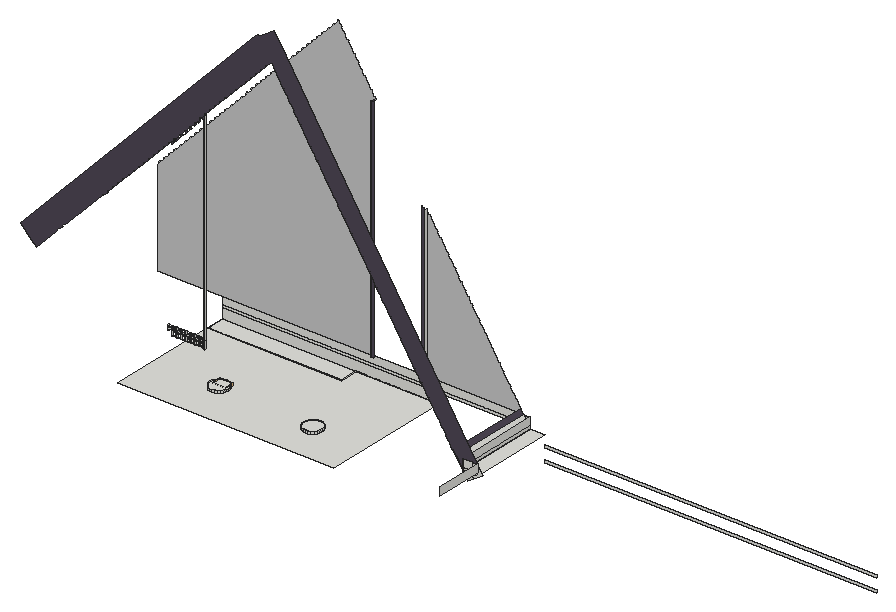
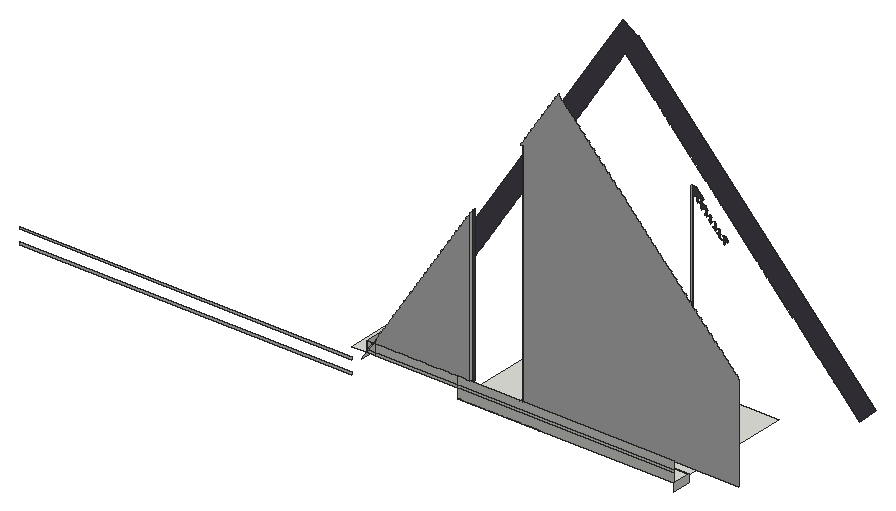
# SketchUp Ruby script. Lengths in inches.
U = 1.inch
M = Sketchup.active_model
def pt(a) = Geom::Point3d.new(a.map { |v| v * U })
def face(e, loops, mat)
  f = e.add_face(loops[0].map { |a| pt(a) })
  loops[1..].each { |l| e.add_face(l.map { |a| pt(a) }).erase! }
  f.material = f.back_material = mat if mat
  f
end
# faces: each face lists its corners as indices into pts; further lists are holes
def faces(e, pts, list, mat = nil) = list.each { |f| face(e, (f[0].is_a?(Array) ? f : [f]).map { |l| l.map { |i| pts[i] } }, mat) }
# xy, xz, yz: faces in a plane at the given z, y or x. An outline is a flat list of corners, or four numbers for a rectangle; further outlines are holes
def ring(l) = l.size == 4 ? [[l[0], l[1]], [l[2], l[1]], [l[2], l[3]], [l[0], l[3]]] : l.each_slice(2).to_a
def flat(e, list, mat, &to3) = list.each { |f| face(e, (f[0].is_a?(Array) ? f : [f]).map { |l| ring(l).map { |u, v| to3.(u, v) } }, mat) }
def xy(e, z, list, mat = nil) = flat(e, list, mat) { |x, y| [x, y, z] }
def xz(e, y, list, mat = nil) = flat(e, list, mat) { |x, z| [x, y, z] }
def yz(e, x, list, mat = nil) = flat(e, list, mat) { |y, z| [x, y, z] }
def lines(e, pts, list) = list.each { |a, b| e.add_line(pt(pts[a]), pt(pts[b])) }
# prism: a flat outline (further loops are holes) pulled along v
def prism(e, loops, v, mat = nil)
  f = face(e, loops, mat); d = Geom::Vector3d.new(v.map { |x| x * U })
  f.pushpull(f.normal.samedirection?(d) ? d.length : -d.length)
end
def box(e, o, s, mat = nil) = prism(e, [[o, [o[0] + s[0], o[1], o[2]], [o[0] + s[0], o[1] + s[1], o[2]], [o[0], o[1] + s[1], o[2]]]], [0, 0, s[2]], mat)
def at(x, y, z, deg = 0) = Geom::Transformation.translation(pt([x, y, z])) * Geom::Transformation.rotation(ORIGIN, Z_AXIS, deg.degrees)
def axes(o, x, y, z) = Geom::Transformation.new([*x, 0, *y, 0, *z, 0, *pt(o).to_a, 1])
def part(name) = M.definitions.add(name)
# library, detail: a bought-in or finely detailed component or shape, given as its bounding box
def library(name, o, s) = part(name).tap { |d| box(d.entities, o, s) }
def detail(e, o, s) = box(e.add_group.entities, o, s)
def put(e, d, t, mat = nil) = e.add_instance(d, t).tap { |i| i.material = mat if mat }
def group(e, t, mat = nil) = e.add_group.tap { |g| g.transformation = t; g.material = mat if mat }.entities
root = M.entities
M.materials.add("[Color M02]").color = [198, 198, 198]
M.materials.add("[Color M06]").color = [79, 71, 84]
c1 = library("A$C06767DEF\#1",[-8.3,1.21,0],[7.09,7.09,5.51])
xy(root,250.875,[[[997.28,2289.06,997.28,2361.68,1083.76,2361.68,1083.76,2373.56,1137.16,2373.56,1137.16,2289.06],[1103.19,2308.39,1104.75,2308.59,1106.19,2309.19,1107.4375,2310.15,1108.39,2311.39,1108.99,2312.84,1109.19,2314.39,1108.99,2315.94,1108.39,2317.39,1107.4375,2318.63,1106.19,2319.58,1104.75,2320.18,1103.19,2320.39,1101.64,2320.18,1100.19,2319.58,1098.95,2318.63,1098,2317.39,1097.4,2315.94,1097.19,2314.39,1097.4,2312.84,1098,2311.39,1098.95,2310.15,1100.19,2309.19,1101.64,2308.59],[1040.12,2311.39,1041.67,2311.59,1043.12,2312.19,1044.36,2313.15,1045.3125,2314.39,1045.91,2315.84,1046.12,2317.39,1045.91,2318.94,1045.3125,2320.39,1044.36,2321.63,1043.12,2322.58,1041.67,2323.18,1040.12,2323.39,1038.5625,2323.18,1037.12,2322.58,1035.875,2321.63,1034.92,2320.39,1034.32,2318.94,1034.12,2317.39,1034.32,2315.84,1034.92,2314.39,1035.875,2313.15,1037.12,2312.19,1038.5625,2311.59]]])
xy(root,251.0625,[[997.28,2361.68,1083.76,2373.56]])
xy(root,252.25,[[1103.19,2308.39,1101.64,2308.59,1100.19,2309.19,1098.95,2310.15,1098,2311.39,1097.4,2312.84,1097.19,2314.39,1097.4,2315.94,1098,2317.39,1098.95,2318.63,1100.19,2319.58,1101.64,2320.18,1103.19,2320.39,1104.75,2320.18,1106.19,2319.58,1107.4375,2318.63,1108.39,2317.39,1108.99,2315.94,1109.19,2314.39,1108.99,2312.84,1108.39,2311.39,1107.4375,2310.15,1106.19,2309.19,1104.75,2308.59]])
xy(root,252.375,[[1040.12,2311.39,1038.5625,2311.59,1037.12,2312.19,1035.875,2313.15,1034.92,2314.39,1034.32,2315.84,1034.12,2317.39,1034.32,2318.94,1034.92,2320.39,1035.875,2321.63,1037.12,2322.58,1038.5625,2323.18,1040.12,2323.39,1041.67,2323.18,1043.12,2322.58,1044.36,2321.63,1045.3125,2320.39,1045.91,2318.94,1046.12,2317.39,1045.91,2315.84,1045.3125,2314.39,1044.36,2313.15,1043.12,2312.19,1041.67,2311.59]])
xy(root,257.0625,[[1196.26,2319.18,1205.57,2373.56]])
xy(root,259.68,[[998.06,2332.13,1000.37,2332.76],[1000.97,2332.13,1003.28,2332.76],[1003.88,2332.13,1006.2,2332.76],[1006.79,2332.13,1009.11,2332.76],[1009.71,2332.13,1012.02,2332.76],
  [1012.62,2332.13,1014.93,2332.76],[1015.53,2332.13,1017.84,2332.76]])
xy(root,262,[[995.15,2332.13,997.46,2332.76],[998.06,2332.13,1000.37,2332.76],[1000.97,2332.13,1003.28,2332.76],[1003.88,2332.13,1006.2,2332.76],[1006.79,2332.13,1009.11,2332.76],
  [1009.71,2332.13,1012.02,2332.76],[1012.62,2332.13,1014.93,2332.76],[1015.53,2332.13,1017.84,2332.76]])
xy(root,262.73,[[995.18,2332.13,997.49,2332.76],[998.09,2332.13,1000.4,2332.76],[1001,2332.13,1003.3125,2332.76],[1003.91,2332.13,1006.22,2332.76],[1006.82,2332.13,1009.14,2332.76],
  [1009.74,2332.13,1012.05,2332.76],[1012.65,2332.13,1014.96,2332.76],[1015.56,2332.13,1017.87,2332.76]])
xy(root,263.89,[[1095.04,2371.68,1096.79,2373.56],[1127.76,2371.68,1129.63,2373.56]])
xy(root,265.04,[[995.18,2332.13,997.49,2332.76],[998.09,2332.13,1000.4,2332.76],[1001,2332.13,1003.3125,2332.76],[1003.91,2332.13,1006.22,2332.76],[1006.82,2332.13,1009.14,2332.76],
  [1009.74,2332.13,1012.05,2332.76],[1012.65,2332.13,1014.96,2332.76],[1015.56,2332.13,1017.87,2332.76]])
xz(root,2319.18,[[1199.5,252.01,1203.55,254.61,1201.98,257.0625,1196.26,257.0625],[1203.55,254.61,1208.8125,257.98,1205.57,263.03,1205.57,257.0625,1201.98,257.0625],[1196.26,257.0625,1201.98,258.95],[1201.98,257.0625,1205.57,258.95],[1196.26,258.95,1201.98,263.89],
  [1201.98,258.95,1205.57,258.95,1205.57,263.03,1205.03,263.89,1201.98,263.89],[1205.57,263.03,1205.03,263.89,1205.57,263.89]])
xz(root,2319.18,[[1196.26,257.0625,1196.26,263.89,1205.03,263.89,1081.6,456.41,1073.92,468.38,1068.66,465.01,1064.27,462.19,1063.71,462.72,1062.38,461.31,910.18,299.61,917.71,292.52,920.85,289.56,923.27,292.13,924.15,293.0625,926.57,295.64,927.45,296.57,929.87,299.14,930.75,300.07,933.17,302.64,934.05,303.58,933.82,303.79,936.24,306.36,936.47,306.15,937.35,307.08,937.12,307.29,939.54,309.87,939.77,309.65,940.64,310.59,943.07,313.16,943.94,314.09,946.36,316.66,947.24,317.59,949.66,320.17,950.54,321.1,952.96,323.67,953.84,324.6,956.26,327.17,957.14,328.11,959.56,330.68,960.4375,331.61,962.86,334.18,963.73,335.11,964.1875,334.6875,966.61,337.26,966.16,337.6875,967.03,338.62,967.49,338.19,969.91,340.76,969.45,341.19,970.33,342.125,970.79,341.69,973.21,344.27,972.75,344.7,973.63,345.63,974.08,345.2,976.51,347.77,976.05,348.2,976.93,349.13,977.38,348.7,979.8,351.28,979.35,351.7,980.23,352.64,980.68,352.21,983.1,354.78,982.65,355.21,983.53,356.14,983.98,355.71,986.4,358.28,985.95,358.71,986.82,359.64,987.28,359.22,989.7,361.79,989.25,362.22,990.12,363.15,990.58,362.72,993,365.29,992.54,365.72,993.42,366.65,993.875,366.22,996.3,368.8,995.84,369.23,996.72,370.16,997.17,369.73,999.6,372.3,999.14,372.73,1000.02,373.66,1000.47,373.23,1002.89,375.81,1002.4375,376.23,1003.32,377.17,1003.77,376.74,1006.19,379.31,1005.74,379.74,1006.62,380.67,1007.07,380.24,1009.49,382.8125,1009.04,383.24,1009.91,384.17,1010.37,383.75,1012.79,386.32,1012.33,386.75,1013.21,387.68,1013.67,387.25,1016.09,389.82,1015.63,390.25,1016.51,391.18,1016.97,390.75,1019.39,393.33,1018.93,393.75,1019.81,394.6875,1020.26,394.26,1022.6875,396.83,1022.23,397.26,1023.11,398.19,1023.5625,397.76,1025.98,400.34,1025.53,400.76,1026.41,401.7,1026.86,401.27,1029.28,403.84,1028.83,404.27,1029.71,405.2,1030.16,404.77,1032.58,407.34,1032.125,407.77,1033,408.7,1033.46,408.28,1035.88,410.85,1035.42,411.28,1036.3,412.21,1036.76,411.78,1039.18,414.35,1038.72,414.78,1039.6,415.71,1040.06,415.28,1042.48,417.86,1042.02,418.28,1042.9,419.22,1043.35,418.79,1045.78,421.36,1045.32,421.79,1046.2,422.72,1046.65,422.29,1049.07,424.86,1048.62,425.29,1049.5,426.23,1049.95,425.8,1052.37,428.37,1051.92,428.8,1052.79,429.73,1053.25,429.3,1055.67,431.875,1055.22,432.3,1056.09,433.23,1056.55,432.81,1058.97,435.38,1058.51,435.81,1059.39,436.74,1059.85,436.31,1062.27,438.88,1061.8125,439.31,1062.69,440.24,1063.15,439.8125,1065.57,442.39,1065.11,442.8125,1065.99,443.75,1066.44,443.32,1068.87,445.89,1068.41,446.32,1069.29,447.25,1069.74,446.82,1072.16,449.39,1071.71,449.82,1071.98,450.11,1071.92,450.2,1072.29,450.4375,1073.86,447.99,1074.35,447.21,1073.99,446.98,1075.68,444.33,1076.05,444.57,1076.55,443.79,1076.18,443.56,1077.875,440.91,1078.24,441.15,1078.74,440.375,1078.37,440.14,1080.07,437.49,1080.43,437.73,1080.93,436.95,1080.5625,436.72,1082.26,434.07,1082.625,434.31,1083.125,433.53,1082.76,433.3,1084.45,430.65,1084.82,430.89,1085.32,430.11,1084.95,429.88,1086.64,427.23,1087.01,427.47,1087.51,426.69,1087.14,426.46,1088.84,423.8125,1089.2,424.05,1089.7,423.27,1089.33,423.04,1091.03,420.39,1091.4,420.63,1091.9,419.85,1091.53,419.62,1093.22,416.97,1093.59,417.21,1094.09,416.43,1093.72,416.2,1095.41,413.55,1095.78,413.79,1096.28,413.01,1095.91,412.78,1097.61,410.13,1097.97,410.37,1098.47,409.59,1098.1,409.36,1099.8,406.71,1100.17,406.95,1100.67,406.17,1100.3,405.9375,1101.99,403.29,1102.36,403.53,1102.86,402.75,1102.49,402.52,1104.18,399.875,1104.55,400.11,1105.05,399.33,1104.68,399.1,1106.375,396.45,1106.75,396.69,1107.24,395.91,1106.875,395.68,1108.57,393.03,1108.9375,393.27,1109.4375,392.49,1109.07,392.26,1110.76,389.61,1111.13,389.85,1111.63,389.07,1111.26,388.84,1112.95,386.19,1113.32,386.43,1113.82,385.65,1113.45,385.42,1115.15,382.77,1115.52,383.01,1116.01,382.23,1115.65,382,1117.34,379.35,1117.71,379.59,1118.21,378.8125,1117.84,378.58,1119.53,375.93,1119.9,376.17,1120.4,375.39,1120.03,375.16,1121.72,372.51,1122.09,372.75,1122.59,371.97,1122.22,371.74,1123.92,369.09,1124.29,369.33,1124.92,368.34,1124.55,368.11,1126.25,365.46,1126.61,365.7,1127.25,364.71,1128.94,362.07,1129.57,361.08,1129.21,360.85,1130.9,358.2,1131.27,358.4375,1131.9,357.45,1131.53,357.22,1133.23,354.57,1133.6,354.81,1134.23,353.82,1133.86,353.58,1135.56,350.94,1135.92,351.18,1136.56,350.19,1136.1875,349.95,1137.88,347.3125,1138.25,347.55,1138.88,346.56,1138.52,346.32,1140.21,343.68,1140.58,343.92,1141.21,342.93,1140.84,342.69,1142.54,340.05,1142.91,340.29,1143.4375,339.46,1143.07,339.22,1144.76,336.58,1145.13,336.8125,1145.66,335.98,1145.3,335.75,1146.99,333.11,1147.36,333.34,1147.89,332.51,1147.52,332.28,1149.22,329.63,1149.59,329.87,1150.12,329.04,1149.75,328.8,1151.44,326.16,1151.8125,326.4,1152.34,325.57,1151.98,325.33,1153.67,322.6875,1154.04,322.92,1154.57,322.09,1154.2,321.86,1155.9,319.21,1156.26,319.45,1156.8,318.62,1156.43,318.38,1158.12,315.74,1158.49,315.98,1159.02,315.15,1158.65,314.91,1160.35,312.27,1160.72,312.51,1161.25,311.68,1160.88,311.44,1162.57,308.8,1162.94,309.03,1163.47,308.2,1163.11,307.97,1164.8,305.32,1165.17,305.56,1165.7,304.73,1165.33,304.49,1167.03,301.85,1167.4,302.09,1167.93,301.26,1167.66,301.09,1169.36,298.45,1169.62,298.61,1170.15,297.79,1169.89,297.62,1171.59,294.97,1171.85,295.14,1172.38,294.3125,1172.12,294.14,1173.8125,291.5,1174.07,291.67,1174.61,290.84,1174.34,290.67,1176.04,288.03,1176.3,288.2,1176.83,287.37,1176.57,287.2,1178.26,284.56,1178.53,284.72,1179.06,283.89,1178.8,283.73,1180.49,281.08,1180.75,281.25,1181.29,280.42,1181.02,280.25,1182.72,277.61,1182.98,277.78,1183.51,276.95,1183.25,276.78,1184.94,274.14,1185.21,274.31,1185.74,273.48,1185.48,273.31,1187.17,270.67,1187.43,270.83,1187.96,270,1187.7,269.84,1189.4,267.19,1189.66,267.36,1190.19,266.53,1189.93,266.36,1191.62,263.72,1191.89,263.89]],"[Color M06]")
xz(root,2332.13,[[1018.44,258.95,1019.02,263.89],[995.18,262.73,997.49,263.89],[998.09,262.73,1000.4,263.89],[1001,262.73,1003.3125,263.89],[1003.91,262.73,1006.22,263.89],
  [1006.82,262.73,1009.14,263.89],[1009.74,262.73,1012.05,263.89],[1012.65,262.73,1014.96,263.89],[1015.56,262.73,1017.87,263.89]])
xz(root,2332.13,[[1018.44,263.89,1019.02,263.89,1019.02,397.75,1016.77,397.75,1011.26,391.9,1012.48,391.9,1012.48,390.44,1013.08,391.08,1013.08,391.9,1015.4,391.9,1015.4,389.59,1013.08,389.59,1013.08,391.08,1012.48,390.44,1012.48,389.59,1011.68,389.59,1011.27,389.15,1010.28,389.15,1010.17,389.03,1010.17,387.98,1009.57,387.35,1009.57,386.84,1009.09,386.84,1008.68,386.4,1009.57,386.4,1009.57,384.09,1007.26,384.09,1007.26,384.89,1006.66,384.25,1006.66,384.09,1006.5,384.09,1006.09,383.65,1006.66,383.65,1006.66,381.34,1004.35,381.34,1004.35,381.8,1003.5,380.9,1003.75,380.9,1003.75,378.59,1001.43,378.59,1001.43,378.7,1000.83,378.07,1000.83,375.84,998.74,375.84,997.92,374.97,997.92,373.09,996.15,373.09,997.92,374.97,997.92,375.4,997.27,375.4,995.61,373.625,995.61,373.09,996.15,373.09,995.68,372.59,997.92,372.59,997.92,370.47,998.52,371.11,998.52,372.59,999.91,372.59,1000.38,373.09,998.52,373.09,998.52,375.4,1000.83,375.4,1000.83,373.57,1001.43,374.21,1001.43,375.4,1002.55,375.4,1002.96,375.84,1001.43,375.84,1001.43,378.15,1003.75,378.15,1003.75,376.68,1004.35,377.32,1004.35,378.15,1005.125,378.15,1005.53,378.59,1004.35,378.59,1004.35,380.9,1006.66,380.9,1006.66,379.79,1007.26,380.43,1007.26,380.9,1007.7,380.9,1008.11,381.34,1007.26,381.34,1007.26,383.65,1009.57,383.65,1009.57,382.89,1010.17,383.53,1010.17,383.65,1010.28,383.65,1010.37,383.75,1010.69,384.09,1010.17,384.09,1010.17,386.4,1012.48,386.4,1012.48,386,1013.27,386.84,1013.08,386.84,1013.08,389.15,1015.4,389.15,1015.4,389.11,1015.99,389.75,1015.99,391.9,1018.01,391.9,1018.44,392.36]],"[Color M06]")
xz(root,2332.76,[[995.18,262.73,997.49,263.89],[998.09,262.73,1000.4,263.89],[1001,262.73,1003.3125,263.89],[1003.91,262.73,1006.22,263.89],[1006.82,262.73,1009.14,263.89],
  [1009.74,262.73,1012.05,263.89],[1012.65,262.73,1014.96,263.89],[1015.56,262.73,1017.87,263.89]])
xz(root,2361.68,[[997.28,250.875,1083.76,251.0625]])
xz(root,2371.68,[[1095.04,263.89,1096.79,412.22],[1127.76,263.89,1129.63,263.89,1129.63,360.99,1129.26,360.76,1129.21,360.85,1129.57,361.08,1128.94,362.07,1128.57,361.83,1127.76,363.11]],"[Color M06]")
xz(root,2373.56,[[1205.57,240.88,1419.96,242.34],[1205.57,249.61,1419.96,251.0625],[1083.76,250.875,1137.16,251.0625],[997.28,251.0625,1137.16,257.0625],[997.28,257.0625,1137.16,258.95],
  [1137.16,257.0625,1190.19,258.95],[1190.19,257.0625,1196.26,257.0625,1195.05,258.95,1190.19,258.95],[1196.26,257.0625,1195.05,258.95,1196.26,258.95],[997.28,258.95,1137.16,263.89],[1137.16,258.95,1190.19,263.89],
  [1190.19,258.95,1195.05,258.95,1191.89,263.89,1191.62,263.72,1191.51,263.89,1190.19,263.89],[1195.05,258.95,1191.89,263.89,1195.05,263.89],[1195.05,258.95,1196.26,263.89],[1191.62,263.72,1191.51,263.89,1191.89,263.89]])
xz(root,2373.56,[[955.23,263.89,1095.04,263.89,1095.04,412.22,1096.27,412.22,1095.97,412.6875,1096.34,412.92,1095.78,413.79,1095.41,413.55,1094.23,415.41,1093.78,416.11,1094.14,416.34,1093.59,417.21,1093.22,416.97,1092.03,418.83,1091.58,419.53,1091.95,419.76,1091.4,420.63,1091.03,420.39,1089.84,422.25,1089.39,422.95,1089.76,423.18,1089.2,424.05,1088.84,423.8125,1087.65,425.67,1087.2,426.37,1087.57,426.6,1087.01,427.47,1086.64,427.23,1085.46,429.09,1085.01,429.79,1085.375,430.02,1084.82,430.89,1084.45,430.65,1083.26,432.51,1082.8125,433.21,1083.18,433.44,1082.625,434.31,1082.26,434.07,1081.07,435.93,1080.62,436.63,1080.99,436.86,1080.43,437.73,1080.07,437.49,1078.88,439.35,1078.43,440.05,1078.8,440.28,1078.24,441.15,1077.875,440.91,1076.69,442.77,1076.24,443.47,1076.6,443.7,1076.05,444.57,1075.68,444.33,1074.49,446.1875,1074.04,446.89,1074.41,447.125,1073.86,447.99,1073.49,447.75,1072.3,449.61,1071.98,450.11,1071.71,449.82,1072.16,449.39,1069.74,446.82,1069.29,447.25,1068.41,446.32,1068.87,445.89,1066.44,443.32,1065.99,443.75,1065.11,442.8125,1065.57,442.39,1063.15,439.8125,1062.69,440.24,1061.8125,439.31,1062.27,438.88,1059.85,436.31,1059.39,436.74,1058.51,435.81,1058.97,435.38,1056.55,432.81,1056.09,433.23,1055.22,432.3,1055.67,431.875,1053.25,429.3,1052.79,429.73,1051.92,428.8,1052.37,428.37,1049.95,425.8,1049.5,426.23,1048.62,425.29,1049.07,424.86,1046.65,422.29,1046.2,422.72,1045.32,421.79,1045.78,421.36,1043.35,418.79,1042.9,419.22,1042.02,418.28,1042.48,417.86,1040.06,415.28,1039.6,415.71,1038.72,414.78,1039.18,414.35,1036.76,411.78,1036.3,412.21,1035.42,411.28,1035.88,410.85,1033.46,408.28,1033,408.7,1032.125,407.77,1032.58,407.34,1030.16,404.77,1029.71,405.2,1028.83,404.27,1029.28,403.84,1026.86,401.27,1026.41,401.7,1025.53,400.76,1025.98,400.34,1023.5625,397.76,1023.11,398.19,1022.23,397.26,1022.6875,396.83,1020.26,394.26,1019.81,394.6875,1018.93,393.75,1019.39,393.33,1016.97,390.75,1016.51,391.18,1015.63,390.25,1016.09,389.82,1013.67,387.25,1013.21,387.68,1012.33,386.75,1012.79,386.32,1010.37,383.75,1009.91,384.17,1009.04,383.24,1009.49,382.8125,1007.07,380.24,1006.62,380.67,1005.74,379.74,1006.19,379.31,1003.77,376.74,1003.32,377.17,1002.4375,376.23,1002.89,375.81,1000.47,373.23,1000.02,373.66,999.14,372.73,999.6,372.3,997.17,369.73,996.72,370.16,995.84,369.23,996.3,368.8,993.875,366.22,993.42,366.65,992.54,365.72,993,365.29,990.58,362.72,990.12,363.15,989.25,362.22,989.7,361.79,987.28,359.22,986.82,359.64,985.95,358.71,986.4,358.28,983.98,355.71,983.53,356.14,982.65,355.21,983.1,354.78,980.68,352.21,980.23,352.64,979.35,351.7,979.8,351.28,977.38,348.7,976.93,349.13,976.05,348.2,976.51,347.77,974.08,345.2,973.63,345.63,972.75,344.7,973.21,344.27,970.79,341.69,970.33,342.125,969.45,341.19,969.91,340.76,969.31,340.125,968.91,339.7,967.49,338.19,967.03,338.62,966.16,337.6875,966.61,337.26,964.1875,334.6875,963.73,335.11,962.86,334.18,963.3125,333.75,960.89,331.18,960.4375,331.61,959.56,330.68,960.01,330.25,957.59,327.68,957.14,328.11,956.26,327.17,956.71,326.75,955.6875,325.65,955.23,325.17],[1129.63,263.89,1190.19,263.89,1190.19,265.95,1189.93,266.36,1190.19,266.53,1189.66,267.36,1189.4,267.19,1187.7,269.84,1187.96,270,1187.43,270.83,1187.17,270.67,1185.48,273.31,1185.74,273.48,1185.21,274.31,1184.94,274.14,1183.25,276.78,1183.51,276.95,1182.98,277.78,1182.72,277.61,1181.02,280.25,1181.29,280.42,1180.75,281.25,1180.49,281.08,1178.8,283.73,1179.06,283.89,1178.53,284.72,1178.26,284.56,1176.57,287.2,1176.83,287.37,1176.3,288.2,1176.04,288.03,1174.34,290.67,1174.61,290.84,1174.07,291.67,1173.8125,291.5,1172.12,294.14,1172.38,294.3125,1171.85,295.14,1171.59,294.97,1169.89,297.62,1170.15,297.79,1169.62,298.61,1169.36,298.45,1167.66,301.09,1167.93,301.26,1167.4,302.09,1167.03,301.85,1165.33,304.49,1165.7,304.73,1165.17,305.56,1164.8,305.32,1163.11,307.97,1163.47,308.2,1162.94,309.03,1162.57,308.8,1160.88,311.44,1161.25,311.68,1160.72,312.51,1160.35,312.27,1158.65,314.91,1159.02,315.15,1158.49,315.98,1158.12,315.74,1156.43,318.38,1156.8,318.62,1156.26,319.45,1155.9,319.21,1154.2,321.86,1154.57,322.09,1154.04,322.92,1153.67,322.6875,1151.98,325.33,1152.34,325.57,1151.8125,326.4,1151.44,326.16,1149.75,328.8,1150.12,329.04,1149.59,329.87,1149.22,329.63,1147.52,332.28,1147.89,332.51,1147.36,333.34,1146.99,333.11,1145.3,335.75,1145.66,335.98,1145.13,336.8125,1144.76,336.58,1143.07,339.22,1143.4375,339.46,1143.01,340.125,1142.91,340.29,1142.54,340.05,1140.84,342.69,1141.21,342.93,1140.58,343.92,1140.21,343.68,1138.52,346.32,1138.88,346.56,1138.25,347.55,1137.88,347.3125,1136.1875,349.95,1136.56,350.19,1135.92,351.18,1135.56,350.94,1133.86,353.58,1134.23,353.82,1133.6,354.81,1133.23,354.57,1131.53,357.22,1131.9,357.45,1131.27,358.4375,1130.9,358.2,1129.63,360.18]],"[Color M02]")
yz(root,997.28,[[2361.68,246.25,2373.56,251.0625]])
yz(root,997.46,[[2332.13,259.68,2332.76,262]])
yz(root,997.49,[[2332.13,262.73,2332.76,265.04]])
yz(root,998.06,[[2332.13,259.68,2332.76,262]])
yz(root,998.09,[[2332.13,262.73,2332.76,265.04]])
yz(root,1000.37,[[2332.13,259.68,2332.76,262]])
yz(root,1000.4,[[2332.13,262.73,2332.76,265.04]])
yz(root,1000.97,[[2332.13,259.68,2332.76,262]])
yz(root,1001,[[2332.13,262.73,2332.76,265.04]])
yz(root,1003.28,[[2332.13,259.68,2332.76,262]])
yz(root,1003.3125,[[2332.13,262.73,2332.76,265.04]])
yz(root,1003.88,[[2332.13,259.68,2332.76,262]])
yz(root,1003.91,[[2332.13,262.73,2332.76,265.04]])
yz(root,1006.2,[[2332.13,259.68,2332.76,262]])
yz(root,1006.22,[[2332.13,262.73,2332.76,265.04]])
yz(root,1006.79,[[2332.13,259.68,2332.76,262]])
yz(root,1006.82,[[2332.13,262.73,2332.76,265.04]])
yz(root,1009.11,[[2332.13,259.68,2332.76,262]])
yz(root,1009.14,[[2332.13,262.73,2332.76,265.04]])
yz(root,1009.71,[[2332.13,259.68,2332.76,262]])
yz(root,1009.74,[[2332.13,262.73,2332.76,265.04]])
yz(root,1012.02,[[2332.13,259.68,2332.76,262]])
yz(root,1012.05,[[2332.13,262.73,2332.76,265.04]])
yz(root,1012.62,[[2332.13,259.68,2332.76,262]])
yz(root,1012.65,[[2332.13,262.73,2332.76,265.04]])
yz(root,1014.93,[[2332.13,259.68,2332.76,262]])
yz(root,1014.96,[[2332.13,262.73,2332.76,265.04]])
yz(root,1015.53,[[2332.13,259.68,2332.76,262]])
yz(root,1015.56,[[2332.13,262.73,2332.76,265.04]])
yz(root,1017.84,[[2332.13,259.68,2332.76,262]])
yz(root,1017.87,[[2332.13,262.73,2332.76,265.04]])
yz(root,1019.02,[[2332.13,258.95,2332.76,263.89],[2332.13,263.89,2332.76,397.75]])
yz(root,1083.76,[[2361.68,250.875,2373.56,251.0625]])
yz(root,1095.04,[[2371.68,263.89,2373.56,412.22]],"[Color M06]")
yz(root,1129.63,[[2371.68,263.89,2373.56,360.99]])
yz(root,1196.26,[[2319.18,257.0625,2373.56,258.95],[2319.18,258.95,2373.56,263.89]])
yz(root,1205.57,[[2289.06,258.95,2319.18,263.89]])
p = [[1103.19,2308.39,250.875],[1101.64,2308.59,250.875],[1101.64,2308.59,252.25],[1103.19,2308.39,252.25],[1104.75,2308.59,250.875],[1104.75,2308.59,252.25],
  [1100.19,2309.19,250.875],[1100.19,2309.19,252.25],[1106.19,2309.19,250.875],[1106.19,2309.19,252.25],[1098.95,2310.15,250.875],[1098.95,2310.15,252.25],
  [1107.4375,2310.15,250.875],[1107.4375,2310.15,252.25],[1098,2311.39,250.875],[1098,2311.39,252.25],[1108.39,2311.39,250.875],[1108.39,2311.39,252.25],
  [1040.12,2311.39,250.875],[1038.5625,2311.59,250.875],[1038.5625,2311.59,252.375],[1040.12,2311.39,252.375],[1041.67,2311.59,250.875],[1041.67,2311.59,252.375],
  [1097.4,2312.84,250.875],[1097.4,2312.84,252.25],[1108.99,2312.84,250.875],[1108.99,2312.84,252.25],[1037.12,2312.19,250.875],[1037.12,2312.19,252.375],
  [1043.12,2312.19,250.875],[1043.12,2312.19,252.375],[1035.875,2313.15,250.875],[1035.875,2313.15,252.375],[1044.36,2313.15,250.875],[1044.36,2313.15,252.375],
  [1097.19,2314.39,250.875],[1097.19,2314.39,252.25],[1109.19,2314.39,250.875],[1109.19,2314.39,252.25],[1034.92,2314.39,250.875],[1034.92,2314.39,252.375],
  [1045.3125,2314.39,250.875],[1045.3125,2314.39,252.375],[1034.32,2315.84,250.875],[1034.32,2315.84,252.375],[1045.91,2315.84,250.875],[1045.91,2315.84,252.375],
  [1097.4,2315.94,250.875],[1097.4,2315.94,252.25],[1108.99,2315.94,250.875],[1108.99,2315.94,252.25],[1034.12,2317.39,250.875],[1034.12,2317.39,252.375],
  [1046.12,2317.39,250.875],[1046.12,2317.39,252.375],[1098,2317.39,250.875],[1098,2317.39,252.25],[1108.39,2317.39,250.875],[1108.39,2317.39,252.25],
  [1034.32,2318.94,250.875],[1034.32,2318.94,252.375],[1045.91,2318.94,250.875],[1045.91,2318.94,252.375],[1098.95,2318.63,250.875],[1098.95,2318.63,252.25],
  [1107.4375,2318.63,250.875],[1107.4375,2318.63,252.25],[1100.19,2319.58,250.875],[1100.19,2319.58,252.25],[1106.19,2319.58,250.875],[1106.19,2319.58,252.25],
  [1034.92,2320.39,250.875],[1034.92,2320.39,252.375],[1045.3125,2320.39,250.875],[1045.3125,2320.39,252.375],[1101.64,2320.18,250.875],[1101.64,2320.18,252.25],
  [1104.75,2320.18,250.875],[1104.75,2320.18,252.25],[1103.19,2320.39,250.875],[1103.19,2320.39,252.25],[1035.875,2321.63,250.875],[1035.875,2321.63,252.375],
  [1044.36,2321.63,250.875],[1044.36,2321.63,252.375],[1037.12,2322.58,250.875],[1037.12,2322.58,252.375],[1043.12,2322.58,250.875],[1043.12,2322.58,252.375],
  [1038.5625,2323.18,250.875],[1038.5625,2323.18,252.375],[1041.67,2323.18,250.875],[1041.67,2323.18,252.375],[1040.12,2323.39,250.875],[1040.12,2323.39,252.375],
  [1196.26,2319.18,257.0625],[1196.26,2373.56,257.0625],[1199.5,2373.56,252.01],[1199.5,2319.18,252.01],[1191.89,2319.18,263.89],[1191.89,2373.56,263.89],
  [1195.05,2373.56,258.95],[1189.93,2373.56,266.36],[1190.19,2373.56,265.95],[1191.51,2373.56,263.89],[1191.62,2373.56,263.72],[1191.62,2319.18,263.72],
  [1189.93,2319.18,266.36]]
faces(root,p,[[0,1,2,3],[4,0,3,5],[1,6,7,2],[8,4,5,9],[6,10,11,7],[12,8,9,13],[10,14,15,11],[16,12,13,17],
  [18,19,20,21],[22,18,21,23],[14,24,25,15],[26,16,17,27],[19,28,29,20],[30,22,23,31],[28,32,33,29],[34,30,31,35],
  [24,36,37,25],[38,26,27,39],[32,40,41,33],[42,34,35,43],[40,44,45,41],[46,42,43,47],[36,48,49,37],[50,38,39,51],
  [44,52,53,45],[54,46,47,55],[48,56,57,49],[58,50,51,59],[52,60,61,53],[62,54,55,63],[56,64,65,57],[66,58,59,67],
  [64,68,69,65],[70,66,67,71],[60,72,73,61],[74,62,63,75],[68,76,77,69],[78,70,71,79],[76,80,81,77],[80,78,79,81],
  [72,82,83,73],[84,74,75,85],[82,86,87,83],[88,84,85,89],[86,90,91,87],[92,88,89,93],[90,94,95,91],[94,92,93,95],
  [96,97,98,99],[96,100,101,102,97],[101,100,107,106]])
faces(root,p,[[103,104,105,106,107,108]],"[Color M06]")
put(root,c1,axes([1045.72,2316.16,249.52],[1.14885,0,0],[0,0.84644,0],[0,0,0.5175]))
put(root,c1,axes([1109.78,2310.37,248.02],[1.14885,0,0],[0,0.84644,0],[0,0,0.5175]))
